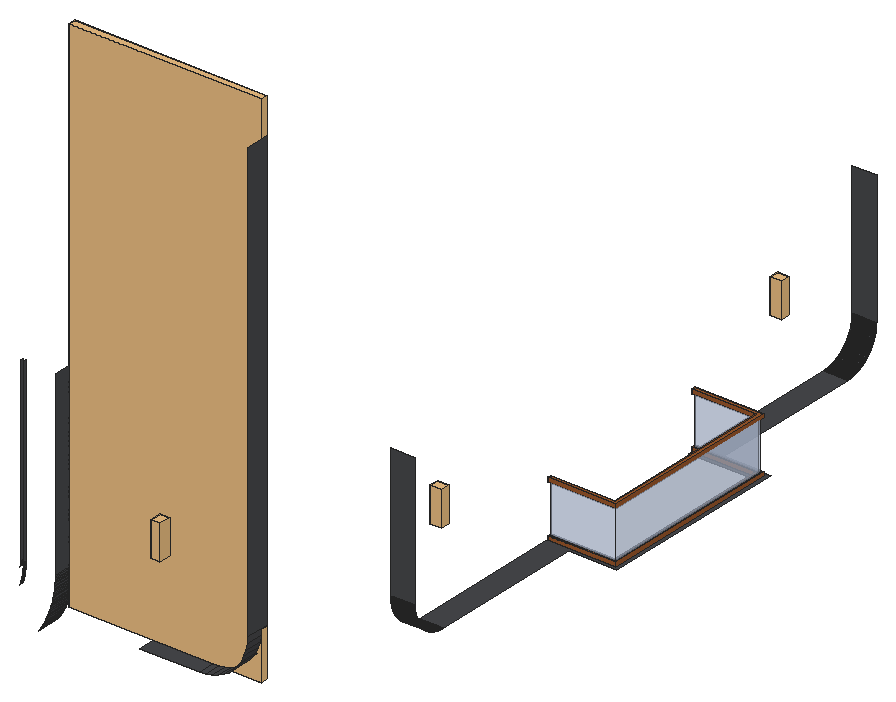
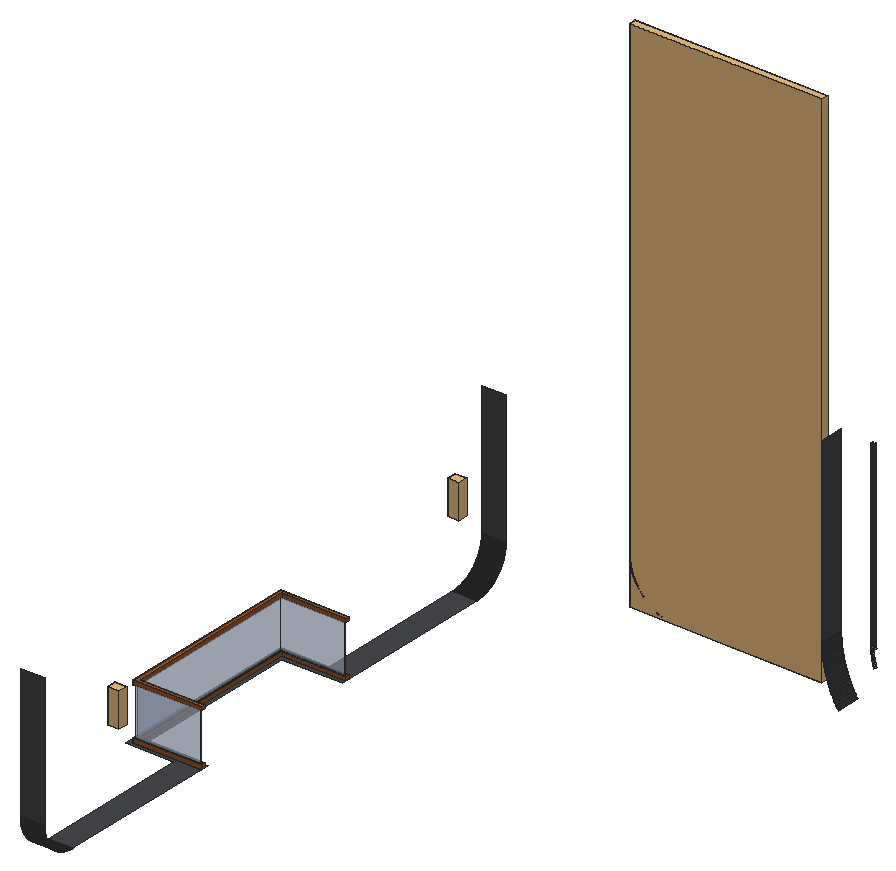
# SketchUp Ruby script. Lengths in inches.
U = 1.inch
M = Sketchup.active_model
def pt(a) = Geom::Point3d.new(a.map { |v| v * U })
def face(e, loops, mat)
  f = e.add_face(loops[0].map { |a| pt(a) })
  loops[1..].each { |l| e.add_face(l.map { |a| pt(a) }).erase! }
  f.material = f.back_material = mat if mat
  f
end
# faces: each face lists its corners as indices into pts; further lists are holes
def faces(e, pts, list, mat = nil) = list.each { |f| face(e, (f[0].is_a?(Array) ? f : [f]).map { |l| l.map { |i| pts[i] } }, mat) }
# xy, xz, yz: faces in a plane at the given z, y or x. An outline is a flat list of corners, or four numbers for a rectangle; further outlines are holes
def ring(l) = l.size == 4 ? [[l[0], l[1]], [l[2], l[1]], [l[2], l[3]], [l[0], l[3]]] : l.each_slice(2).to_a
def flat(e, list, mat, &to3) = list.each { |f| face(e, (f[0].is_a?(Array) ? f : [f]).map { |l| ring(l).map { |u, v| to3.(u, v) } }, mat) }
def xy(e, z, list, mat = nil) = flat(e, list, mat) { |x, y| [x, y, z] }
def xz(e, y, list, mat = nil) = flat(e, list, mat) { |x, z| [x, y, z] }
def yz(e, x, list, mat = nil) = flat(e, list, mat) { |y, z| [x, y, z] }
def lines(e, pts, list) = list.each { |a, b| e.add_line(pt(pts[a]), pt(pts[b])) }
# prism: a flat outline (further loops are holes) pulled along v
def prism(e, loops, v, mat = nil)
  f = face(e, loops, mat); d = Geom::Vector3d.new(v.map { |x| x * U })
  f.pushpull(f.normal.samedirection?(d) ? d.length : -d.length)
end
def box(e, o, s, mat = nil) = prism(e, [[o, [o[0] + s[0], o[1], o[2]], [o[0] + s[0], o[1] + s[1], o[2]], [o[0], o[1] + s[1], o[2]]]], [0, 0, s[2]], mat)
def at(x, y, z, deg = 0) = Geom::Transformation.translation(pt([x, y, z])) * Geom::Transformation.rotation(ORIGIN, Z_AXIS, deg.degrees)
def axes(o, x, y, z) = Geom::Transformation.new([*x, 0, *y, 0, *z, 0, *pt(o).to_a, 1])
def part(name) = M.definitions.add(name)
# library, detail: a bought-in or finely detailed component or shape, given as its bounding box
def library(name, o, s) = part(name).tap { |d| box(d.entities, o, s) }
def detail(e, o, s) = box(e.add_group.entities, o, s)
def put(e, d, t, mat = nil) = e.add_instance(d, t).tap { |i| i.material = mat if mat }
def group(e, t, mat = nil) = e.add_group.tap { |g| g.transformation = t; g.material = mat if mat }.entities
root = M.entities
M.materials.add("1432 AP 8245 TAR ROAD").color = [71, 72, 75]
M.materials.add("Outer Light").color = [251, 217, 152]
M.materials.add("[Translucent Glass Blue]").color = [195, 208, 233]
M.materials["[Translucent Glass Blue]"].alpha = 0.5
M.materials.add("[Wood Cherry Original]").color = [152, 86, 42]
M.materials.add("[Wood Veneer 01]").color = [120, 70, 37]
c1 = library("WALL LIGHT 69",[4.19,4.05,-8.78],[4.61,5.7,17.13])
c2 = library("Group\#15",[0,-3.5,0],[96,3.5,261])
c3 = part("Group\#47")
xy(c3.entities,0,[[0,0,0,2,32,2,32,90,0,90,0,92,34,92,34,0]])
xy(c3.entities,1.75,[[0.75,0.75,33.25,0.75,33.25,91.25,0.75,91.25,0.75,90.75,32.75,90.75,32.75,1.25,0.75,1.25]])
xy(c3.entities,2,[[[0,0,34,0,34,92,0,92,0,90,32,90,32,2,0,2],[0.75,0.75,0.75,1.25,32.75,1.25,32.75,90.75,0.75,90.75,0.75,91.25,33.25,91.25,33.25,0.75]]])
xy(c3.entities,26,[[[0,0,0,2,32,2,32,90,0,90,0,92,34,92,34,0],[0.75,0.75,33.25,0.75,33.25,91.25,0.75,91.25,0.75,90.75,32.75,90.75,32.75,1.25,0.75,1.25]]])
xy(c3.entities,26.25,[[0.75,0.75,0.75,1.25,32.75,1.25,32.75,90.75,0.75,90.75,0.75,91.25,33.25,91.25,33.25,0.75]])
xy(c3.entities,28,[[0,0,34,0,34,92,0,92,0,90,32,90,32,2,0,2]])
xz(c3.entities,0,[[0,0,34,2],[0,26,34,28]])
xz(c3.entities,0.75,[[0.75,1.75,33.25,2],[0.75,26,33.25,26.25]])
xz(c3.entities,1.25,[[0.75,1.75,32.75,2],[0.75,26,32.75,26.25]])
xz(c3.entities,2,[[0,0,32,2],[0,26,32,28]])
xz(c3.entities,90,[[0,0,32,2],[0,26,32,28]])
xz(c3.entities,90.75,[[0.75,1.75,32.75,2],[0.75,26,32.75,26.25]])
xz(c3.entities,91.25,[[0.75,1.75,33.25,2],[0.75,26,33.25,26.25]])
xz(c3.entities,92,[[0,0,34,2],[0,26,34,28]])
yz(c3.entities,0,[[0,0,2,2],[90,0,92,2],[0,26,2,28],[90,26,92,28]])
yz(c3.entities,0.75,[[0.75,1.75,1.25,2],[90.75,1.75,91.25,2],[0.75,26,1.25,26.25],[90.75,26,91.25,26.25]])
yz(c3.entities,32,[[2,0,90,2],[2,26,90,28]])
yz(c3.entities,32.75,[[1.25,1.75,90.75,2],[1.25,26,90.75,26.25]])
yz(c3.entities,33.25,[[0.75,1.75,91.25,2],[0.75,26,91.25,26.25]])
yz(c3.entities,34,[[0,0,92,2],[0,26,92,28]])
g1 = group(c3.entities,at(0.75,0.75,1.75),"[Translucent Glass Blue]")
prism(g1,[[[32,90,0],[0,90,0],[0,90.5,0],[32.5,90.5,0],[32.5,0,0],[0,0,0],[0,0.5,0],[32,0.5,0]]],[0,0,24.5])
xy(root,302.79,[[486,95.37,516,107.37]],"1432 AP 8245 TAR ROAD")
xy(root,317.79,[[573,161.13,585,161.37],[573,161.37,585,161.37,585,239.37,609,239.37,609,335.37,585,335.37,585,413.37,573,413.37,573,329.37,603,329.37,603,245.37,573,245.37],[573,413.37,585,413.61]],"1432 AP 8245 TAR ROAD")
xz(root,143.37,[[573,335.56,585,335.79],[573,335.79,585,401.79]],"1432 AP 8245 TAR ROAD")
xz(root,431.36,[[573,335.09,585,335.32]],"1432 AP 8245 TAR ROAD")
xz(root,431.37,[[573,335.56,585,335.79],[573,335.79,585,401.79]],"1432 AP 8245 TAR ROAD")
yz(root,426.5,[[95.37,320.35,96.87,320.79],[95.37,320.79,96.87,410.79]],"1432 AP 8245 TAR ROAD")
yz(root,426.5,[[95.37,320.35,96.87,320.79],[95.37,320.79,96.87,410.79]],"Outer Light")
yz(root,428,[[95.37,320.33,96.87,320.79],[95.37,320.79,96.87,410.79]],"1432 AP 8245 TAR ROAD")
yz(root,428,[[95.37,320.33,96.87,320.79],[95.37,320.79,96.87,410.79]],"Outer Light")
yz(root,444,[[95.37,320.125,107.37,320.79],[95.37,320.79,107.37,410.79]],"1432 AP 8245 TAR ROAD")
yz(root,540,[[95.37,326.79,107.37,545.79]],"1432 AP 8245 TAR ROAD")
p = [[435.77,107.37,293.02],[436.13,107.37,293.58],[436.13,95.37,293.58],[435.77,95.37,293.02],[436.48,107.37,294.14],[436.48,95.37,294.14],
  [436.83,107.37,294.72],[436.83,95.37,294.72],[437.17,107.37,295.29],[437.17,95.37,295.29],[437.5,107.37,295.87],[437.5,95.37,295.87],
  [437.82,107.37,296.46],[437.82,95.37,296.46],[438.13,107.37,297.05],[438.13,95.37,297.05],[438.44,107.37,297.64],[438.44,95.37,297.64],
  [438.74,107.37,298.24],[438.74,95.37,298.24],[439.03,107.37,298.84],[439.03,95.37,298.84],[439.32,107.37,299.44],[439.32,95.37,299.44],
  [439.59,107.37,300.05],[439.59,95.37,300.05],[439.86,107.37,300.66],[439.86,95.37,300.66],[440.12,107.37,301.28],[440.12,95.37,301.28],
  [440.37,107.37,301.89],[440.37,95.37,301.89],[440.61,107.37,302.52],[440.61,95.37,302.52],[440.85,107.37,303.14],[440.85,95.37,303.14],
  [516,95.37,302.79],[519.13,95.37,303],[519.13,107.37,303],[516,107.37,302.79],[522.21,95.37,303.61],[522.21,107.37,303.61],
  [441.07,107.37,303.77],[441.07,95.37,303.77],[525.18,95.37,304.62],[525.18,107.37,304.62],[441.29,107.37,304.4],[441.29,95.37,304.4],
  [441.5,107.37,305.03],[441.5,95.37,305.03],[528,95.37,306.01],[528,107.37,306.01],[441.71,107.37,305.67],[441.71,95.37,305.67],
  [441.9,107.37,306.31],[441.9,95.37,306.31],[530.61,95.37,307.75],[530.61,107.37,307.75],[442.09,107.37,306.95],[442.09,95.37,306.95],
  [442.26,107.37,307.59],[442.26,95.37,307.59],[442.43,107.37,308.24],[442.43,95.37,308.24],[532.97,95.37,309.82],[532.97,107.37,309.82],
  [442.59,107.37,308.89],[442.59,95.37,308.89],[442.74,107.37,309.54],[442.74,95.37,309.54],[442.89,107.37,310.1875],[442.89,95.37,310.1875],
  [535.04,95.37,312.18],[535.04,107.37,312.18],[443.02,107.37,310.84],[443.02,95.37,310.84],[426.43,95.37,310.41],[426.56,95.37,310.85],
  [426.56,96.87,310.85],[426.43,96.87,310.41],[426.43,96.87,310.41],[426.56,96.87,310.85],[426.56,95.37,310.85],[426.43,95.37,310.41],
  [443.15,107.37,311.5],[443.15,95.37,311.5],[426.6875,95.37,311.29],[426.6875,96.87,311.29],[426.6875,96.87,311.29],[426.6875,95.37,311.29],
  [426.81,95.37,311.73],[426.81,96.87,311.73],[426.81,96.87,311.73],[426.81,95.37,311.73],[443.26,107.37,312.16],[443.26,95.37,312.16],
  [426.92,95.37,312.18],[426.92,96.87,312.18],[426.92,96.87,312.18],[426.92,95.37,312.18],[427.03,95.37,312.62],[427.03,96.87,312.62],
  [427.03,96.87,312.62],[427.03,95.37,312.62],[443.37,107.37,312.8125],[443.37,95.37,312.8125],[536.78,95.37,314.79],[536.78,107.37,314.79],
  [427.14,95.37,313.07],[427.14,96.87,313.07],[427.14,96.87,313.07],[427.14,95.37,313.07],[443.47,107.37,313.47],[443.47,95.37,313.47],
  [427.24,95.37,313.52],[427.24,96.87,313.52],[427.24,96.87,313.52],[427.24,95.37,313.52],[427.33,95.37,313.96],[427.33,96.87,313.96],
  [427.33,96.87,313.96],[427.33,95.37,313.96],[443.5625,107.37,314.14],[443.5625,95.37,314.14],[427.41,95.37,314.41],[427.41,96.87,314.41],
  [427.41,96.87,314.41],[427.41,95.37,314.41],[443.65,107.37,314.8],[443.65,95.37,314.8],[427.49,95.37,314.86],[427.49,96.87,314.86],
  [427.49,96.87,314.86],[427.49,95.37,314.86],[443.72,107.37,315.46],[443.72,95.37,315.46],[538.17,95.37,317.61],[538.17,107.37,317.61],
  [427.57,95.37,315.32],[427.57,96.87,315.32],[427.57,96.87,315.32],[427.57,95.37,315.32],[427.64,95.37,315.77],[427.64,96.87,315.77],
  [427.64,96.87,315.77],[427.64,95.37,315.77],[443.79,107.37,316.125],[443.79,95.37,316.125],[427.7,95.37,316.22],[427.7,96.87,316.22],
  [427.7,96.87,316.22],[427.7,95.37,316.22],[443.84,107.37,316.79],[443.84,95.37,316.79],[427.76,95.37,316.68],[427.76,96.87,316.68],
  [427.76,96.87,316.68],[427.76,95.37,316.68],[427.81,95.37,317.13],[427.81,96.87,317.13],[427.81,96.87,317.13],[427.81,95.37,317.13],
  [443.89,107.37,317.46],[443.89,95.37,317.46],[427.85,95.37,317.59],[427.85,96.87,317.59],[427.85,96.87,317.59],[427.85,95.37,317.59],
  [443.93,107.37,318.12],[443.93,95.37,318.12],[427.89,95.37,318.05],[427.89,96.87,318.05],[427.89,96.87,318.05],[427.89,95.37,318.05],
  [539.18,95.37,320.58],[539.18,107.37,320.58],[573,159.96,317.85],[573,159.72,317.87],[585,159.72,317.87],[585,159.96,317.85],
  [573,160.19,317.83],[585,160.19,317.83],[573,160.43,317.82],[585,160.43,317.82],[573,160.66,317.81],[585,160.66,317.81],
  [573,160.9,317.8],[585,160.9,317.8],[573,161.13,317.79],[585,161.13,317.79],[573,413.84,317.8],[573,413.61,317.79],
  [585,413.61,317.79],[585,413.84,317.8],[573,414.08,317.81],[585,414.08,317.81],[573,414.3125,317.82],[585,414.3125,317.82],
  [573,414.55,317.83],[585,414.55,317.83],[573,414.78,317.85],[585,414.78,317.85],[573,415.02,317.87],[585,415.02,317.87],
  [573,159.02,317.95],[573,158.79,317.98],[585,158.79,317.98],[585,159.02,317.95],[573,159.25,317.92],[585,159.25,317.92],
  [573,159.49,317.89],[585,159.49,317.89],[573,415.25,317.89],[585,415.25,317.89],[573,415.49,317.92],[585,415.49,317.92],
  [573,415.72,317.95],[585,415.72,317.95],[573,415.95,317.98],[585,415.95,317.98],[427.93,95.37,318.5],[427.93,96.87,318.5],
  [427.93,96.87,318.5],[427.93,95.37,318.5],[573,158.55,318.01],[573,158.32,318.05],[585,158.32,318.05],[585,158.55,318.01],
  [573,416.1875,318.01],[585,416.1875,318.01],[573,416.42,318.05],[585,416.42,318.05],[443.96,107.37,318.79],[443.96,95.37,318.79],
  [573,157.86,318.14],[573,157.63,318.19],[585,157.63,318.19],[585,157.86,318.14],[573,158.09,318.09],[585,158.09,318.09],
  [573,416.65,318.09],[585,416.65,318.09],[573,416.88,318.14],[585,416.88,318.14],[573,417.11,318.19],[585,417.11,318.19],
  [573,157.4,318.24],[573,157.17,318.29],[585,157.17,318.29],[585,157.4,318.24],[573,417.34,318.24],[585,417.34,318.24],
  [573,417.57,318.29],[585,417.57,318.29],[573,156.9375,318.35],[573,156.71,318.41],[585,156.71,318.41],[585,156.9375,318.35],
  [573,417.8,318.35],[585,417.8,318.35],[573,418.03,318.41],[585,418.03,318.41],[573,156.48,318.47],[585,156.48,318.47],
  [573,418.26,318.47],[585,418.26,318.47],[427.95,95.37,318.96],[427.95,96.87,318.96],[427.95,96.87,318.96],[427.95,95.37,318.96],
  [573,156.26,318.53],[573,156.03,318.6],[585,156.03,318.6],[585,156.26,318.53],[573,418.48,318.53],[585,418.48,318.53],
  [573,418.71,318.6],[585,418.71,318.6],[426.45,96.87,319.04],[426.43,96.87,318.6],[426.43,95.37,318.6],[426.45,95.37,319.04],
  [426.45,95.37,319.04],[426.43,95.37,318.6],[426.43,96.87,318.6],[426.45,96.87,319.04],[573,155.81,318.67],[585,155.81,318.67],
  [573,418.93,318.67],[585,418.93,318.67],[573,155.58,318.75],[573,155.36,318.82],[585,155.36,318.82],[585,155.58,318.75],
  [573,419.16,318.75],[585,419.16,318.75],[573,419.38,318.82],[585,419.38,318.82],[443.98,107.37,319.46],[443.98,95.37,319.46],
  [573,155.14,318.9],[585,155.14,318.9],[573,419.6,318.9],[585,419.6,318.9],[573,154.92,318.99],[585,154.92,318.99],
  [573,419.82,318.99],[585,419.82,318.99],[426.47,96.87,319.48],[426.47,95.37,319.48],[426.47,95.37,319.48],[426.47,96.87,319.48],
  [427.97,95.37,319.42],[427.97,96.87,319.42],[427.97,96.87,319.42],[427.97,95.37,319.42],[573,154.7,319.07],[585,154.7,319.07],
  [573,420.04,319.07],[585,420.04,319.07],[573,154.48,319.16],[585,154.48,319.16],[573,420.26,319.16],[585,420.26,319.16],
  [573,154.26,319.25],[585,154.26,319.25],[573,420.48,319.25],[585,420.48,319.25],[573,154.05,319.35],[573,153.83,319.45],
  [585,153.83,319.45],[585,154.05,319.35],[573,420.69,319.35],[585,420.69,319.35],[573,420.91,319.45],[585,420.91,319.45],
  [427.99,95.37,319.875],[427.99,96.87,319.875],[427.99,96.87,319.875],[427.99,95.37,319.875],[573,153.62,319.55],[585,153.62,319.55],
  [573,421.12,319.55],[585,421.12,319.55],[426.49,96.87,319.92],[426.49,95.37,319.92],[426.49,95.37,319.92],[426.49,96.87,319.92],
  [444,107.37,320.125],[444,95.37,320.125],[573,153.41,319.65],[585,153.41,319.65],[573,421.33,319.65],[585,421.33,319.65],
  [573,153.2,319.75],[585,153.2,319.75],[573,421.54,319.75],[585,421.54,319.75],[573,152.99,319.86],[585,152.99,319.86],
  [573,421.75,319.86],[585,421.75,319.86],[426.5,96.87,320.35],[426.5,95.37,320.35],[426.5,95.37,320.35],[426.5,96.87,320.35],
  [428,95.37,320.33],[428,96.87,320.33],[428,96.87,320.33],[428,95.37,320.33],[573,152.78,319.97],[585,152.78,319.97],
  [573,421.96,319.97],[585,421.96,319.97],[573,152.57,320.09],[585,152.57,320.09],[573,422.17,320.09],[585,422.17,320.09],
  [573,152.37,320.2],[585,152.37,320.2],[573,422.37,320.2],[585,422.37,320.2],[573,152.17,320.32],[585,152.17,320.32],
  [573,422.57,320.32],[585,422.57,320.32],[573,151.96,320.44],[585,151.96,320.44],[573,422.77,320.44],[585,422.77,320.44],
  [573,151.76,320.57],[585,151.76,320.57],[573,422.97,320.57],[585,422.97,320.57],[539.79,95.37,323.66],[539.79,107.37,323.66],
  [573,151.57,320.7],[585,151.57,320.7],[573,423.17,320.7],[585,423.17,320.7],[573,151.37,320.83],[585,151.37,320.83],
  [573,423.37,320.83],[585,423.37,320.83],[573,151.17,320.96],[585,151.17,320.96],[573,423.57,320.96],[585,423.57,320.96],
  [573,150.98,321.09],[585,150.98,321.09],[573,423.76,321.09],[585,423.76,321.09],[573,150.79,321.23],[585,150.79,321.23],
  [573,423.95,321.23],[585,423.95,321.23],[573,150.6,321.37],[585,150.6,321.37],[573,424.14,321.37],[585,424.14,321.37],
  [573,150.41,321.51],[585,150.41,321.51],[573,424.33,321.51],[585,424.33,321.51],[573,150.23,321.66],[585,150.23,321.66],
  [573,424.51,321.66],[585,424.51,321.66],[573,150.04,321.8],[585,150.04,321.8],[573,424.7,321.8],[585,424.7,321.8],
  [573,149.86,321.95],[585,149.86,321.95],[573,424.88,321.95],[585,424.88,321.95],[573,149.68,322.1],[585,149.68,322.1],
  [573,425.06,322.1],[585,425.06,322.1],[573,149.5,322.26],[585,149.5,322.26],[573,425.24,322.26],[585,425.24,322.26],
  [573,149.33,322.42],[585,149.33,322.42],[573,425.41,322.42],[585,425.41,322.42],[573,149.15,322.57],[585,149.15,322.57],
  [573,425.59,322.57],[585,425.59,322.57],[573,148.98,322.74],[585,148.98,322.74],[573,425.76,322.74],[585,425.76,322.74],
  [573,148.81,322.9],[585,148.81,322.9],[573,425.93,322.9],[585,425.93,322.9],[573,148.64,323.0625],[585,148.64,323.0625],
  [573,426.1,323.0625],[585,426.1,323.0625],[573,148.48,323.23],[585,148.48,323.23],[573,426.26,323.23],[585,426.26,323.23],
  [573,148.3125,323.4],[585,148.3125,323.4],[573,426.43,323.4],[585,426.43,323.4],[573,148.15,323.57],[585,148.15,323.57],
  [573,426.59,323.57],[585,426.59,323.57],[573,147.99,323.75],[585,147.99,323.75],[573,426.75,323.75],[585,426.75,323.75],
  [540,95.37,326.79],[540,107.37,326.79],[573,147.84,323.92],[585,147.84,323.92],[573,426.9,323.92],[585,426.9,323.92],
  [573,147.68,324.1],[585,147.68,324.1],[573,427.06,324.1],[585,427.06,324.1],[573,147.53,324.28],[585,147.53,324.28],
  [573,427.21,324.28],[585,427.21,324.28],[573,147.38,324.46],[585,147.38,324.46],[573,427.36,324.46],[585,427.36,324.46],
  [573,147.23,324.65],[585,147.23,324.65],[573,427.51,324.65],[585,427.51,324.65],[573,147.09,324.83],[585,147.09,324.83],
  [573,427.65,324.83],[585,427.65,324.83],[573,146.95,325.02],[585,146.95,325.02],[573,427.79,325.02],[585,427.79,325.02],
  [573,146.81,325.21],[585,146.81,325.21],[573,427.93,325.21],[585,427.93,325.21],[573,146.67,325.4],[585,146.67,325.4],
  [573,428.07,325.4],[585,428.07,325.4],[573,146.54,325.6],[585,146.54,325.6],[573,428.2,325.6],[585,428.2,325.6],
  [573,146.4,325.79],[585,146.4,325.79],[573,428.34,325.79],[585,428.34,325.79],[573,146.27,325.99],[585,146.27,325.99],
  [573,428.47,325.99],[585,428.47,325.99],[573,146.15,326.1875],[585,146.15,326.1875],[573,428.59,326.1875],[585,428.59,326.1875],
  [573,146.02,326.39],[585,146.02,326.39],[573,428.72,326.39],[585,428.72,326.39],[573,145.9,326.59],[585,145.9,326.59],
  [573,428.84,326.59],[585,428.84,326.59],[573,145.78,326.79],[585,145.78,326.79],[573,428.96,326.79],[585,428.96,326.79],
  [573,145.67,327],[585,145.67,327],[573,429.07,327],[585,429.07,327],[573,145.55,327.2],[585,145.55,327.2],
  [573,429.1875,327.2],[585,429.1875,327.2],[573,145.44,327.41],[585,145.44,327.41],[573,429.3,327.41],[585,429.3,327.41],
  [573,145.33,327.62],[585,145.33,327.62],[573,429.41,327.62],[585,429.41,327.62],[573,145.23,327.83],[585,145.23,327.83],
  [573,429.51,327.83],[585,429.51,327.83],[573,145.125,328.04],[585,145.125,328.04],[573,429.62,328.04],[585,429.62,328.04],
  [573,145.02,328.26],[585,145.02,328.26],[573,429.72,328.26],[585,429.72,328.26],[573,144.93,328.47],[585,144.93,328.47],
  [573,429.8125,328.47],[585,429.8125,328.47],[573,144.83,328.6875],[585,144.83,328.6875],[573,429.91,328.6875],[585,429.91,328.6875],
  [573,144.74,328.9],[585,144.74,328.9],[573,430,328.9],[585,430,328.9],[573,144.65,329.12],[585,144.65,329.12],
  [573,430.09,329.12],[585,430.09,329.12],[573,144.57,329.34],[585,144.57,329.34],[573,430.17,329.34],[585,430.17,329.34],
  [573,144.48,329.5625],[585,144.48,329.5625],[573,430.26,329.5625],[585,430.26,329.5625],[573,144.4,329.78],[585,144.4,329.78],
  [573,430.34,329.78],[585,430.34,329.78],[573,144.33,330.01],[585,144.33,330.01],[573,430.41,330.01],[585,430.41,330.01],
  [573,144.25,330.23],[585,144.25,330.23],[573,430.49,330.23],[585,430.49,330.23],[573,144.18,330.45],[585,144.18,330.45],
  [573,430.56,330.45],[585,430.56,330.45],[573,144.11,330.68],[585,144.11,330.68],[573,430.63,330.68],[585,430.63,330.68],
  [573,144.05,330.91],[585,144.05,330.91],[573,430.69,330.91],[585,430.69,330.91],[573,143.98,331.13],[585,143.98,331.13],
  [573,430.76,331.13],[585,430.76,331.13],[573,143.92,331.36],[585,143.92,331.36],[573,430.82,331.36],[585,430.82,331.36],
  [573,143.87,331.59],[585,143.87,331.59],[573,430.87,331.59],[585,430.87,331.59],[573,143.8125,331.82],[585,143.8125,331.82],
  [573,430.93,331.82],[585,430.93,331.82],[573,143.76,332.05],[585,143.76,332.05],[573,430.98,332.05],[585,430.98,332.05],
  [573,143.72,332.28],[585,143.72,332.28],[573,431.02,332.28],[585,431.02,332.28],[573,143.67,332.51],[585,143.67,332.51],
  [573,431.07,332.51],[585,431.07,332.51],[573,143.63,332.74],[585,143.63,332.74],[573,431.11,332.74],[585,431.11,332.74],
  [573,143.59,332.98],[585,143.59,332.98],[573,431.15,332.98],[585,431.15,332.98],[573,143.56,333.21],[585,143.56,333.21],
  [573,431.18,333.21],[585,431.18,333.21],[573,143.52,333.44],[585,143.52,333.44],[573,431.22,333.44],[585,431.22,333.44],
  [573,143.49,333.68],[585,143.49,333.68],[573,431.25,333.68],[585,431.25,333.68],[573,143.47,333.91],[585,143.47,333.91],
  [573,431.27,333.91],[585,431.27,333.91],[573,143.45,334.15],[585,143.45,334.15],[573,431.29,334.15],[585,431.29,334.15],
  [573,143.43,334.38],[585,143.43,334.38],[573,431.3125,334.38],[585,431.3125,334.38],[573,143.41,334.61],[585,143.41,334.61],
  [573,431.33,334.61],[585,431.33,334.61],[573,143.39,334.85],[585,143.39,334.85],[573,431.35,334.85],[585,431.35,334.85],
  [573,143.38,335.09],[585,143.38,335.09],[573,431.36,335.09],[585,431.36,335.09],[573,143.375,335.32],[585,143.375,335.32],
  [573,143.37,335.56],[585,143.37,335.56],[573,431.37,335.56],[573,431.36,335.32],[585,431.36,335.32],[585,431.37,335.56]]
faces(root,p,[[0,1,2,3],[1,4,5,2],[4,6,7,5],[6,8,9,7],[8,10,11,9],[10,12,13,11],[12,14,15,13],[14,16,17,15],
  [16,18,19,17],[18,20,21,19],[20,22,23,21],[22,24,25,23],[24,26,27,25],[26,28,29,27],[28,30,31,29],[30,32,33,31],
  [32,34,35,33],[36,37,38,39],[37,40,41,38],[34,42,43,35],[40,44,45,41],[42,46,47,43],[46,48,49,47],[44,50,51,45],
  [48,52,53,49],[52,54,55,53],[50,56,57,51],[54,58,59,55],[58,60,61,59],[60,62,63,61],[56,64,65,57],[62,66,67,63],
  [66,68,69,67],[68,70,71,69],[64,72,73,65],[70,74,75,71],[76,77,78,79],[74,84,85,75],[77,86,87,78],[86,90,91,87],
  [84,94,95,85],[90,96,97,91],[96,100,101,97],[94,104,105,95],[72,106,107,73],[100,108,109,101],[104,112,113,105],[108,114,115,109],
  [114,118,119,115],[112,122,123,113],[118,124,125,119],[122,128,129,123],[124,130,131,125],[128,134,135,129],[106,136,137,107],[130,138,139,131],
  [138,142,143,139],[134,146,147,135],[142,148,149,143],[146,152,153,147],[148,154,155,149],[154,158,159,155],[152,162,163,153],[158,164,165,159],
  [162,168,169,163],[164,170,171,165],[136,174,175,137],[176,177,178,179],[180,176,179,181],[182,180,181,183],[184,182,183,185],[186,184,185,187],
  [188,186,187,189],[190,191,192,193],[194,190,193,195],[196,194,195,197],[198,196,197,199],[200,198,199,201],[202,200,201,203],[204,205,206,207],
  [208,204,207,209],[210,208,209,211],[177,210,211,178],[212,202,203,213],[214,212,213,215],[216,214,215,217],[218,216,217,219],[170,220,221,171],
  [224,225,226,227],[205,224,227,206],[228,218,219,229],[230,228,229,231],[168,232,233,169],[234,235,236,237],[238,234,237,239],[225,238,239,226],
  [240,230,231,241],[242,240,241,243],[244,242,243,245],[246,247,248,249],[235,246,249,236],[250,244,245,251],[252,250,251,253],[254,255,256,257],
  [247,254,257,248],[258,252,253,259],[260,258,259,261],[255,262,263,256],[264,260,261,265],[220,266,267,221],[270,271,272,273],[262,270,273,263],
  [274,264,265,275],[276,274,275,277],[282,283,284,285],[271,286,287,272],[288,276,277,289],[290,291,292,293],[286,290,293,287],[294,288,289,295],
  [296,294,295,297],[232,298,299,233],[291,300,301,292],[302,296,297,303],[300,304,305,301],[306,302,303,307],[310,282,285,311],[266,312,313,267],
  [304,316,317,305],[318,306,307,319],[316,320,321,317],[322,318,319,323],[320,324,325,321],[326,322,323,327],[328,329,330,331],[324,328,331,325],
  [332,326,327,333],[334,332,333,335],[312,336,337,313],[329,340,341,330],[342,334,335,343],[346,310,311,347],[298,348,349,299],[340,350,351,341],
  [352,342,343,353],[350,354,355,351],[356,352,353,357],[354,358,359,355],[360,356,357,361],[364,346,347,365],[336,366,367,337],[358,370,371,359],
  [372,360,361,373],[370,374,375,371],[376,372,373,377],[374,378,379,375],[380,376,377,381],[378,382,383,379],[384,380,381,385],[382,386,387,383],
  [388,384,385,389],[386,390,391,387],[392,388,389,393],[174,394,395,175],[390,396,397,391],[398,392,393,399],[396,400,401,397],[402,398,399,403],
  [400,404,405,401],[406,402,403,407],[404,408,409,405],[410,406,407,411],[408,412,413,409],[414,410,411,415],[412,416,417,413],[418,414,415,419],
  [416,420,421,417],[422,418,419,423],[420,424,425,421],[426,422,423,427],[424,428,429,425],[430,426,427,431],[428,432,433,429],[434,430,431,435],
  [432,436,437,433],[438,434,435,439],[436,440,441,437],[442,438,439,443],[440,444,445,441],[446,442,443,447],[444,448,449,445],[450,446,447,451],
  [448,452,453,449],[454,450,451,455],[452,456,457,453],[458,454,455,459],[456,460,461,457],[462,458,459,463],[460,464,465,461],[466,462,463,467],
  [464,468,469,465],[470,466,467,471],[468,472,473,469],[474,470,471,475],[472,476,477,473],[478,474,475,479],[394,480,481,395],[476,482,483,477],
  [484,478,479,485],[482,486,487,483],[488,484,485,489],[486,490,491,487],[492,488,489,493],[490,494,495,491],[496,492,493,497],[494,498,499,495],
  [500,496,497,501],[498,502,503,499],[504,500,501,505],[502,506,507,503],[508,504,505,509],[506,510,511,507],[512,508,509,513],[510,514,515,511],
  [516,512,513,517],[514,518,519,515],[520,516,517,521],[518,522,523,519],[524,520,521,525],[522,526,527,523],[528,524,525,529],[526,530,531,527],
  [532,528,529,533],[530,534,535,531],[536,532,533,537],[534,538,539,535],[540,536,537,541],[538,542,543,539],[544,540,541,545],[542,546,547,543],
  [548,544,545,549],[546,550,551,547],[552,548,549,553],[550,554,555,551],[556,552,553,557],[554,558,559,555],[560,556,557,561],[558,562,563,559],
  [564,560,561,565],[562,566,567,563],[568,564,565,569],[566,570,571,567],[572,568,569,573],[570,574,575,571],[576,572,573,577],[574,578,579,575],
  [580,576,577,581],[578,582,583,579],[584,580,581,585],[582,586,587,583],[588,584,585,589],[586,590,591,587],[592,588,589,593],[590,594,595,591],
  [596,592,593,597],[594,598,599,595],[600,596,597,601],[598,602,603,599],[604,600,601,605],[602,606,607,603],[608,604,605,609],[606,610,611,607],
  [612,608,609,613],[610,614,615,611],[616,612,613,617],[614,618,619,615],[620,616,617,621],[618,622,623,619],[624,620,621,625],[622,626,627,623],
  [628,624,625,629],[626,630,631,627],[632,628,629,633],[630,634,635,631],[636,632,633,637],[634,638,639,635],[640,636,637,641],[638,642,643,639],
  [644,640,641,645],[642,646,647,643],[648,644,645,649],[646,650,651,647],[652,648,649,653],[650,654,655,651],[656,652,653,657],[654,658,659,655],
  [660,656,657,661],[658,662,663,659],[664,660,661,665],[662,666,667,663],[668,664,665,669],[666,670,671,667],[672,668,669,673],[670,674,675,671],
  [676,672,673,677],[674,678,679,675],[680,676,677,681],[678,682,683,679],[684,680,681,685],[682,686,687,683],[688,684,685,689],[686,690,691,687],
  [692,688,689,693],[690,694,695,691],[694,696,697,695],[698,699,700,701]],"1432 AP 8245 TAR ROAD")
faces(root,p,[[80,81,82,83],[81,88,89,82],[88,92,93,89],[92,98,99,93],[98,102,103,99],[102,110,111,103],[110,116,117,111],[116,120,121,117],
  [120,126,127,121],[126,132,133,127],[132,140,141,133],[140,144,145,141],[144,150,151,145],[150,156,157,151],[156,160,161,157],[160,166,167,161],
  [166,172,173,167],[172,222,223,173],[222,268,269,223],[278,279,280,281],[308,278,281,309],[268,314,315,269],[314,338,339,315],[344,308,309,345],
  [362,344,345,363],[338,368,369,339]],"Outer Light")
put(root,c1,at(485.24,94.12,352.05))
put(root,c2,at(444,107.37,302.79),"[Wood Veneer 01]")
put(root,c1,at(583.25,162.99,366.66,90))
put(root,c1,at(583.25,375.38,366.66,90))
put(root,c3,at(573,241.37,317.79),"[Wood Cherry Original]")
